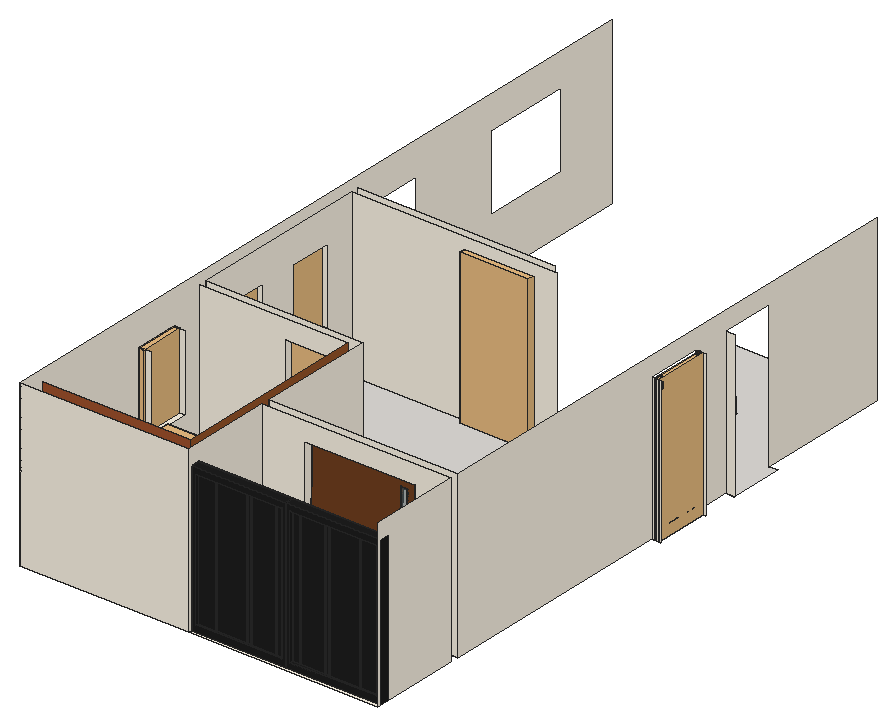
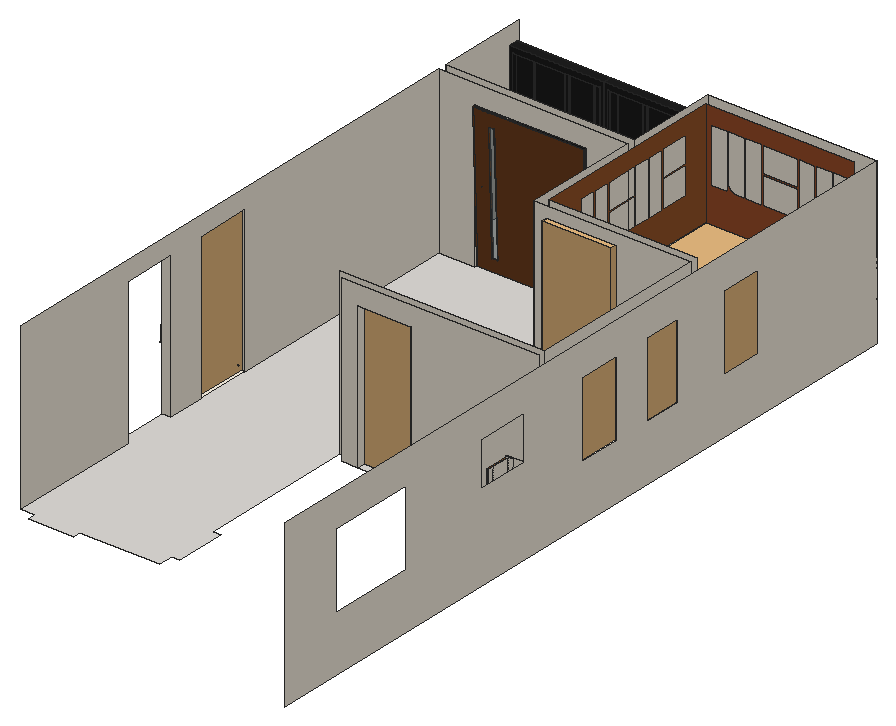
# SketchUp Ruby script. Lengths in inches.
U = 1.inch
M = Sketchup.active_model
def pt(a) = Geom::Point3d.new(a.map { |v| v * U })
def face(e, loops, mat)
  f = e.add_face(loops[0].map { |a| pt(a) })
  loops[1..].each { |l| e.add_face(l.map { |a| pt(a) }).erase! }
  f.material = f.back_material = mat if mat
  f
end
# faces: each face lists its corners as indices into pts; further lists are holes
def faces(e, pts, list, mat = nil) = list.each { |f| face(e, (f[0].is_a?(Array) ? f : [f]).map { |l| l.map { |i| pts[i] } }, mat) }
# xy, xz, yz: faces in a plane at the given z, y or x. An outline is a flat list of corners, or four numbers for a rectangle; further outlines are holes
def ring(l) = l.size == 4 ? [[l[0], l[1]], [l[2], l[1]], [l[2], l[3]], [l[0], l[3]]] : l.each_slice(2).to_a
def flat(e, list, mat, &to3) = list.each { |f| face(e, (f[0].is_a?(Array) ? f : [f]).map { |l| ring(l).map { |u, v| to3.(u, v) } }, mat) }
def xy(e, z, list, mat = nil) = flat(e, list, mat) { |x, y| [x, y, z] }
def xz(e, y, list, mat = nil) = flat(e, list, mat) { |x, z| [x, y, z] }
def yz(e, x, list, mat = nil) = flat(e, list, mat) { |y, z| [x, y, z] }
def lines(e, pts, list) = list.each { |a, b| e.add_line(pt(pts[a]), pt(pts[b])) }
# prism: a flat outline (further loops are holes) pulled along v
def prism(e, loops, v, mat = nil)
  f = face(e, loops, mat); d = Geom::Vector3d.new(v.map { |x| x * U })
  f.pushpull(f.normal.samedirection?(d) ? d.length : -d.length)
end
def box(e, o, s, mat = nil) = prism(e, [[o, [o[0] + s[0], o[1], o[2]], [o[0] + s[0], o[1] + s[1], o[2]], [o[0], o[1] + s[1], o[2]]]], [0, 0, s[2]], mat)
def at(x, y, z, deg = 0) = Geom::Transformation.translation(pt([x, y, z])) * Geom::Transformation.rotation(ORIGIN, Z_AXIS, deg.degrees)
def axes(o, x, y, z) = Geom::Transformation.new([*x, 0, *y, 0, *z, 0, *pt(o).to_a, 1])
def part(name) = M.definitions.add(name)
# library, detail: a bought-in or finely detailed component or shape, given as its bounding box
def library(name, o, s) = part(name).tap { |d| box(d.entities, o, s) }
def detail(e, o, s) = box(e.add_group.entities, o, s)
def put(e, d, t, mat = nil) = e.add_instance(d, t).tap { |i| i.material = mat if mat }
def group(e, t, mat = nil) = e.add_group.tap { |g| g.transformation = t; g.material = mat if mat }.entities
root = M.entities
M.materials.add("Material \#0").color = [86, 53, 35]
M.materials.add("Material \#1").color = [140, 140, 140]
M.materials.add("[0030_OldLace]").color = [253, 245, 230]
M.materials.add("[0040_Peru]").color = [205, 133, 63]
M.materials.add("[0042_Sienna]").color = [160, 82, 45]
M.materials.add("[Color M08]1").color = [30, 30, 30]
M.materials.add("[Metal_Seamed]").color = [118, 119, 115]
M.materials.add("[Terrazzo Tile Accent]").color = [224, 221, 217]
M.materials.add("[Translucent_Glass_Safety]").color = [93, 108, 112]
M.materials["[Translucent_Glass_Safety]"].alpha = 0.5
M.materials.add("[Wood Cherry Original]").color = [152, 86, 42]
M.materials.add("[Wood_Cherry_Original]").color = [112, 63, 31]
M.materials.add("[Wood_Cherry_Original]1").color = [152, 86, 42]
c1 = part("Group\#102")
g1 = group(c1.entities,at(0,0,0))
prism(g1,[[[0,3,72],[70.5,3,72],[70.5,3,0],[0,3,0]],[[67.5,3,3],[67.5,3,69],[3,3,69],[3,3,3]]],[0,-3,0])
c2 = part("Group\#135")
box(c2.entities,[0,0,0],[0.5,1,66])
c3 = part("Framed panel assembly")
g2 = group(c3.entities,at(-446.34,-0.4375,0),"[Color M08]1")
put(g2,c1,axes([69,0,0],[-0.97872,0,0],[0,2.08853,0],[0,0,1.5]))
g3 = group(g2,at(2.9375,4.18,4.5))
g4 = group(g3,at(0,-2.09,0))
box(g4,[0,0,0],[5.39,2.09,99])
box(g4,[49.75,0,0],[13.38,2.09,99])
box(g4,[27.46,0,0],[21.8,2.09,99])
box(g4,[24.13,0,0],[2.84,2.09,99])
box(g4,[5.875,0,0],[17.77,2.09,99])
put(g3,c2,axes([49.26,0,0],[0.97872,0,0],[0,-2.08853,0],[0,0,1.5]))
put(g3,c2,axes([23.65,0,0],[0.97872,0,0],[0,-2.08853,0],[0,0,1.5]))
put(g3,c2,axes([26.97,0,0],[0.97872,0,0],[0,-2.08853,0],[0,0,1.5]))
put(g3,c2,axes([5.39,0,0],[0.97872,0,0],[0,-2.08853,0],[0,0,1.5]))
g5 = group(c3.entities,at(-446.34,-0.4375,0),"[Color M08]1")
put(g5,c1,axes([-69,0,0],[0.97872,0,0],[0,2.08853,0],[0,0,1.5]))
g6 = group(g5,at(-2.9375,4.18,4.5))
g7 = group(g6,at(0,-2.09,0))
box(g7,[-5.39,0,0],[5.39,2.09,99])
box(g7,[-63.13,0,0],[13.38,2.09,99])
box(g7,[-49.26,0,0],[21.8,2.09,99])
box(g7,[-26.97,0,0],[2.84,2.09,99])
box(g7,[-23.65,0,0],[17.77,2.09,99])
put(g6,c2,axes([-49.26,0,0],[-0.97872,0,0],[0,-2.08853,0],[0,0,1.5]))
put(g6,c2,axes([-23.65,0,0],[-0.97872,0,0],[0,-2.08853,0],[0,0,1.5]))
put(g6,c2,axes([-26.97,0,0],[-0.97872,0,0],[0,-2.08853,0],[0,0,1.5]))
put(g6,c2,axes([-5.39,0,0],[-0.97872,0,0],[0,-2.08853,0],[0,0,1.5]))
c4 = library("Group\#25",[0,0,0],[108,114,40.125])
c5 = part("Untitled (1)")
xy(c5.entities,0,[[[-89.01,-44.6,-13.76,84.15],[-78.58,-32.92,-74.95,73.47]]],"[Wood_Cherry_Original]")
xy(c5.entities,2.5,[[-78.58,-32.92,-74.95,73.47]],"[Translucent_Glass_Safety]")
xy(c5.entities,4.25,[[[-89.01,-44.6,-13.76,84.15],[-79.26,-33.6,-74.26,74.15],[-86.22,18.76,-84.6,20.07],[-86.22,-0.43,-84.6,0.51]],[-79.26,-33.6,-74.95,-33.6,-74.95,-32.92,-78.58,-32.92,-78.58,73.47,-74.26,73.47,-74.26,74.15,-79.26,74.15],[-74.95,-33.6,-74.26,73.47]],"[Wood_Cherry_Original]")
xy(c5.entities,5.75,[[-86.22,0.51,-84.6,18.76]],"[Metal_Seamed]")
xy(c5.entities,6.75,[[-86.22,-0.43,-84.6,20.07]],"[Metal_Seamed]")
xz(c5.entities,-44.6,[[-89.01,0,-13.76,4.25]],"[Wood_Cherry_Original]")
xz(c5.entities,-32.92,[[-78.58,0,-74.95,2.5],[-78.58,2.5,-74.95,4.25]],"[Wood_Cherry_Original]")
xz(c5.entities,-0.43,[[-86.22,4.25,-84.6,6.75]],"[Wood_Cherry_Original]")
xz(c5.entities,0.51,[[-86.22,4.25,-84.6,5.75]],"[Metal_Seamed]")
xz(c5.entities,18.76,[[-86.22,4.25,-84.6,5.75]],"[Metal_Seamed]")
xz(c5.entities,20.07,[[-86.22,4.25,-84.6,6.75]],"[Wood_Cherry_Original]")
xz(c5.entities,73.47,[[-78.58,0,-74.95,2.5],[-78.58,2.5,-74.95,4.25]],"[Wood_Cherry_Original]")
xz(c5.entities,84.15,[[-89.01,0,-13.76,4.25]],"[Wood_Cherry_Original]")
yz(c5.entities,-89.01,[[-44.6,0,84.15,4.25]],"[Wood_Cherry_Original]")
yz(c5.entities,-86.22,[[-0.43,4.25,-0.43,6.75,20.07,6.75,20.07,4.25,18.76,4.25,18.76,5.75,0.51,5.75,0.51,4.25]],"[Metal_Seamed]")
yz(c5.entities,-84.6,[[-0.43,4.25,0.51,4.25,0.51,5.75,18.76,5.75,18.76,4.25,20.07,4.25,20.07,6.75,-0.43,6.75]],"[Metal_Seamed]")
yz(c5.entities,-78.58,[[-32.92,2.5,73.47,4.25]],"[Wood_Cherry_Original]")
yz(c5.entities,-78.58,[[-32.92,0,73.47,2.5]],"[Wood_Cherry_Original]1")
yz(c5.entities,-74.95,[[-32.92,0,73.47,2.5],[-32.92,2.5,73.47,4.25]],"[Wood_Cherry_Original]")
yz(c5.entities,-13.76,[[-44.6,0,84.15,4.25]],"[Wood_Cherry_Original]")
c6 = library("Window 82-25",[-14.97,-2.34,0.01],[29.93,4.71,56.48])
c7 = library("Sliding door",[-0.09,-1.01,0],[50.15,5.52,90.11])
c8 = part("3DGeom~18_Defintion")
xz(c8.entities,-241.71,[[-976.3,0,23.7,0,23.7,7.58],[-976.3,0,23.7,7.58,-976.3,7.58]],"Material \#0")
xz(c8.entities,241.71,[[-976.3,0,-976.3,7.58,23.7,7.58],[-976.3,0,23.7,7.58,23.7,0]],"Material \#0")
yz(c8.entities,23.7,[[-241.71,0,0,0,-241.71,7.58],[0,0,0,7.58,-241.71,7.58],[0,0,241.71,0,241.71,7.58],[0,0,241.71,7.58,0,7.58]],"Material \#0")
c9 = part("3DGeom~20_Defintion")
xy(c9.entities,0,[[-976.3,-241.71,-976.3,-223.46,23.7,-241.71],[23.7,-241.71,-976.3,-223.46,5.45,-223.46],[23.7,-241.71,5.45,-223.46,5.45,0],[23.7,-241.71,5.45,0,23.7,0],[-976.3,-223.46,-976.3,-211.85,5.45,-223.46],
  [5.45,-223.46,-976.3,-211.85,-6.16,-211.85],[5.45,-223.46,-6.16,-211.85,-6.16,0],[5.45,-223.46,-6.16,0,5.45,0],[-6.16,0,-6.16,211.85,5.45,223.46],[-6.16,0,5.45,223.46,5.45,0],
  [5.45,0,23.7,241.71,23.7,0],[5.45,0,5.45,223.46,23.7,241.71],[-976.3,211.85,-976.3,223.46,5.45,223.46],[-976.3,211.85,5.45,223.46,-6.16,211.85],[-976.3,223.46,-976.3,241.71,23.7,241.71],
  [-976.3,223.46,23.7,241.71,5.45,223.46]],"Material \#0")
c10 = part("3DGeom~22_Defintion")
xz(c10.entities,-210.625,[[-1016.13,2.47,-1016.13,9.96,-16.28,2.47],[-16.28,2.47,-1016.13,9.96,-16.28,9.96],[-1016.13,9.96,-1016.13,51.7,-16.28,51.7],[-1016.13,9.96,-16.28,51.7,-16.28,9.96],[-1016.13,51.7,-1016.13,72.71,-16.28,51.7]],"Material \#0")
xz(c10.entities,210.625,[[-1016.13,2.47,-16.28,2.47,-1016.13,9.96],[-16.28,2.47,-16.28,9.96,-1016.13,9.96],[-1016.13,9.96,-16.28,51.7,-1016.13,51.7],[-1016.13,9.96,-16.28,9.96,-16.28,51.7],[-1016.13,51.7,-16.28,51.7,-1016.13,72.71]],"Material \#0")
yz(c10.entities,-16.28,[[-210.625,2.47,-210.625,9.96,0,9.96],[-210.625,2.47,0,9.96,0,2.47],[0,2.47,0,9.96,210.625,2.47],[210.625,2.47,0,9.96,210.625,9.96],[-210.625,9.96,-210.625,51.7,0,51.7],
  [-210.625,9.96,0,51.7,0,9.96],[0,9.96,0,51.7,210.625,9.96],[210.625,9.96,0,51.7,210.625,51.7],[-210.625,51.7,0,72.71,0,51.7],[0,51.7,0,72.71,210.625,51.7]],"Material \#0")
p = [[-1016.13,-210.625,72.71],[-16.13,-210.77,73.09],[-16.28,-210.625,51.7],[-16.28,-210.625,51.7],[-16.13,-210.77,73.09],[-16.28,0,72.71],
  [-16.13,210.77,73.09],[-16.28,210.625,51.7],[-16.28,210.625,51.7],[-16.13,210.77,73.09],[-1016.13,210.625,72.71]]
faces(c10.entities,p,[[0,1,2],[3,4,5],[5,6,7],[8,9,10]],"Material \#0")
c11 = part("3DGeom~19_Defintion")
xy(c11.entities,0,[[-6.28,-215.79,-994.45,-208.55,-13.52,-208.55],[-994.45,-215.79,-994.45,-208.55,-6.28,-215.79],[-6.28,-215.79,-13.52,-208.55,-13.52,0],[-6.28,-215.79,-13.52,0,-6.28,0],[-13.52,0,-13.52,208.55,-6.28,215.79],
  [-13.52,0,-6.28,215.79,-6.28,0],[-994.45,208.55,-6.28,215.79,-13.52,208.55],[-994.45,208.55,-994.45,215.79,-6.28,215.79]],"Material \#0")
p = [[-13.52,-208.55,0],[-994.45,-208.55,0],[-994.45,-207.81,0.07],[-14.25,-207.81,0.07],[-13.52,-208.55,0],[-14.25,-207.81,0.07],
  [-14.25,0,0.07],[-13.52,0,0],[-13.52,208.55,0],[-14.25,207.81,0.07],[-13.52,208.55,0],[-14.25,207.81,0.07],
  [-994.45,207.81,0.07],[-994.45,208.55,0],[-994.45,-207.21,0.27],[-994.45,-207.21,0.27],[-14.86,-207.21,0.27],[-14.86,-207.21,0.27],
  [-14.86,0,0.27],[-14.86,0,0.27],[-14.86,0,0.27],[-14.86,0,0.27],[-14.86,207.21,0.27],[-14.86,207.21,0.27],
  [-994.45,207.21,0.27],[-994.45,207.21,0.27],[-14.86,-207.21,0.27],[-994.45,-207.21,0.27],[-994.45,-206.74,0.6],[-15.33,-206.74,0.6],
  [-14.86,-207.21,0.27],[-15.33,-206.74,0.6],[-15.33,0,0.6],[-14.86,0,0.27],[-14.86,207.21,0.27],[-15.33,206.74,0.6],
  [-14.86,207.21,0.27],[-15.33,206.74,0.6],[-994.45,206.74,0.6],[-994.45,207.21,0.27],[-994.45,-206.4,1.07],[-15.66,-206.4,1.07],
  [-15.66,-206.4,1.07],[-15.66,0,1.07],[-15.66,206.4,1.07],[-15.66,206.4,1.07],[-994.45,206.4,1.07],[-994.45,-206.2,1.68],
  [-15.86,-206.2,1.68],[-15.86,-206.2,1.68],[-15.86,0,1.68],[-15.86,206.2,1.68],[-15.86,206.2,1.68],[-994.45,206.2,1.68],
  [-994.45,-206.13,2.41],[-15.93,-206.13,2.41],[-15.93,-206.13,2.41],[-15.93,0,2.41],[-15.93,206.13,2.41],[-15.93,206.13,2.41],
  [-994.45,206.13,2.41],[-994.45,-206.13,71.16],[-994.45,-206.22,71.59],[-15.79,-206.28,71.53],[-15.79,-206.28,71.53],[-15.84,0,71.59],
  [-15.93,0,71.16],[-15.79,206.28,71.53],[-15.79,206.28,71.53],[-994.45,206.22,71.59],[-994.45,206.13,71.16],[-15.79,-206.28,71.53],
  [-994.45,-206.48,71.84],[-994.45,-206.9,71.93],[-15.16,-206.9,71.93],[-15.79,-206.28,71.53],[-15.79,-206.28,71.53],[-15.16,-206.9,71.93],
  [-15.16,0,71.93],[-994.45,-206.48,71.84],[-15.59,0,71.84],[-15.79,-206.28,71.53],[-15.59,0,71.84],[-15.79,206.28,71.53],
  [-15.16,206.9,71.93],[-15.59,0,71.84],[-15.79,206.28,71.53],[-994.45,206.48,71.84],[-15.79,206.28,71.53],[-15.16,206.9,71.93],
  [-994.45,206.9,71.93],[-994.45,206.48,71.84],[-15.79,206.28,71.53],[-994.45,-227.27,72.01],[5.41,-227.47,72.33],[4.78,-226.84,71.93],
  [4.78,-226.84,71.93],[5.41,-227.47,72.33],[5.21,0,72.01],[-994.45,-226.84,71.93],[-994.45,-227.27,72.01],[5.21,0,72.01],
  [4.78,0,71.93],[4.78,226.84,71.93],[5.21,0,72.01],[5.21,0,72.01],[5.41,227.47,72.33],[4.78,226.84,71.93],
  [5.41,227.47,72.33],[-994.45,227.27,72.01],[-994.45,227.27,72.01],[-994.45,226.84,71.93],[-994.45,-227.27,72.01],[-994.45,-227.53,72.27],
  [5.41,-227.47,72.33],[5.41,-227.47,72.33],[5.47,0,72.27],[5.21,0,72.01],[5.41,227.47,72.33],[5.41,227.47,72.33],
  [-994.45,227.53,72.27],[-994.45,227.27,72.01],[-994.45,-227.61,72.7],[-994.45,-227.61,74.4375],[-994.45,-227.61,74.4375],[5.55,-227.61,74.4375],
  [5.55,-227.61,74.4375],[5.55,0,74.4375],[5.55,0,72.7],[5.55,227.61,74.4375],[5.55,227.61,74.4375],[-994.45,227.61,74.4375],
  [-994.45,227.61,74.4375],[-994.45,227.61,72.7]]
faces(c11.entities,p,[[0,1,2],[2,3,0],[4,5,6],[6,7,4],[8,7,6],[6,9,8],[10,11,12],[12,13,10],
  [3,2,14],[15,16,3],[5,17,18],[19,6,5],[9,6,20],[21,22,9],[11,23,24],[25,12,11],
  [26,27,28],[28,29,26],[30,31,32],[32,33,30],[34,33,32],[32,35,34],[36,37,38],[38,39,36],
  [29,28,40],[40,41,29],[31,42,43],[43,32,31],[35,32,43],[43,44,35],[37,45,46],[46,38,37],
  [41,40,47],[47,48,41],[42,49,50],[50,43,42],[44,43,50],[50,51,44],[45,52,53],[53,46,45],
  [48,47,54],[54,55,48],[49,56,57],[57,50,49],[51,50,57],[57,58,51],[52,59,60],[60,53,52],
  [61,62,63],[64,65,66],[66,65,67],[68,69,70],[71,72,73],[73,74,75],[76,77,78],[62,79,63],
  [78,80,76],[81,82,65],[83,80,78],[78,84,83],[65,85,86],[68,87,69],[88,89,90],[90,91,92],
  [93,94,95],[96,97,98],[95,99,100],[101,102,96],[103,102,104],[105,106,103],[107,108,109],[110,111,107],
  [112,113,114],[115,116,117],[117,116,118],[119,120,121],[114,122,123],[124,125,114],[113,122,114],[115,126,127],
  [127,128,115],[115,128,116],[118,128,127],[127,129,118],[116,128,118],[119,130,131],[132,133,119],[119,133,120]],"Material \#0")
c12 = part("3DGeom~15_Defintion")
xy(c12.entities,0,[[-961.58,-251.9,-958.5,-248.8125,-961.58,-237.8],[-961.58,-251.9,28.8,-248.8125,-958.5,-248.8125],[-961.58,-251.9,36.25,-251.9,28.8,-248.8125],[36.25,-251.9,19.98,-239.99,28.8,-248.8125],[36.25,-251.9,22.16,-237.8,19.98,-239.99],
  [-958.5,-248.8125,-958.5,-237.8,-961.58,-237.8],[19.98,-239.99,22.16,-237.8,3.36,-223.37],[-958.5,-237.8,-958.5,-223.37,-961.58,-220.28],[-961.58,-237.8,-958.5,-237.8,-961.58,-220.28],[22.16,-237.8,4.64,-220.28,3.36,-223.37],
  [-958.5,-223.37,4.64,-220.28,-961.58,-220.28],[-958.5,-223.37,3.36,-223.37,4.64,-220.28],[5.29,-219.63,8.375,-218.35,5.29,0],[8.375,-218.35,8.375,0,5.29,0],[5.29,0,8.375,0,5.29,219.63],
  [8.375,0,8.375,218.35,5.29,219.63],[8.375,218.35,22.8125,237.15,5.29,219.63],[-961.58,220.28,-958.5,223.37,-961.58,237.8],[-961.58,220.28,3.36,223.37,-958.5,223.37],[-961.58,220.28,4.64,220.28,3.36,223.37],
  [4.64,220.28,19.98,239.99,3.36,223.37],[4.64,220.28,22.16,237.8,19.98,239.99],[-958.5,223.37,-958.5,237.8,-961.58,237.8],[-958.5,237.8,-958.5,248.8125,-961.58,251.9],[-961.58,237.8,-958.5,237.8,-961.58,251.9],
  [22.16,237.8,28.8,248.8125,19.98,239.99],[22.16,237.8,36.25,251.9,28.8,248.8125],[-958.5,248.8125,36.25,251.9,-961.58,251.9],[-958.5,248.8125,28.8,248.8125,36.25,251.9]],"Material \#0")
xy(c12.entities,7.48,[[-962.79,-238.36,23.37,-238.36,-962.79,-219.67],[23.37,-238.36,4.67,-219.67,-962.79,-219.67],[23.37,-238.36,23.37,0,4.67,-219.67],[4.67,-219.67,23.37,0,4.67,0],[23.37,0,23.37,238.36,4.67,219.67],
  [4.67,0,23.37,0,4.67,219.67],[-962.79,219.67,23.37,238.36,-962.79,238.36],[-962.79,219.67,4.67,219.67,23.37,238.36]],"Material \#0")
xy(c12.entities,63.5625,[[-962.79,-238.36,-962.79,-219.67,4.67,-219.67],[-962.79,-238.36,4.67,-219.67,23.37,-238.36],[23.37,-238.36,4.67,-219.67,23.37,0],[4.67,-219.67,4.67,0,23.37,0],[23.37,0,4.67,219.67,23.37,238.36],
  [4.67,0,4.67,219.67,23.37,0],[-962.79,219.67,-962.79,238.36,4.67,219.67],[4.67,219.67,-962.79,238.36,23.37,238.36]],"Material \#0")
xy(c12.entities,69.64,[[-962.79,-219.62,4.63,-219.62,-962.79,-200.32],[4.63,-219.62,-14.68,-200.32,-962.79,-200.32],[4.63,-219.62,4.63,0,-14.68,-200.32],[-14.68,-200.32,4.63,0,-14.68,0],[-14.68,0,4.63,0,-14.68,200.32],
  [4.63,0,4.63,219.62,-14.68,200.32],[-962.79,200.32,-14.68,200.32,4.63,219.62],[-962.79,200.32,4.63,219.62,-962.79,219.62]],"Material \#0")
xy(c12.entities,71.04,[[-961.58,-251.9,-958.5,-248.8125,28.8,-248.8125],[-961.58,-251.9,-961.58,-237.8,-958.5,-248.8125],[-961.58,-251.9,28.8,-248.8125,36.25,-251.9],[36.25,-251.9,19.98,-239.99,22.16,-237.8],[36.25,-251.9,28.8,-248.8125,19.98,-239.99],
  [-958.5,-248.8125,-961.58,-237.8,-958.5,-237.8],[19.98,-239.99,3.36,-223.37,22.16,-237.8],[-958.5,-237.8,-961.58,-220.28,-958.5,-223.37],[-961.58,-237.8,-961.58,-220.28,-958.5,-237.8],[22.16,-237.8,3.36,-223.37,4.64,-220.28],
  [-958.5,-223.37,-961.58,-220.28,4.64,-220.28],[-958.5,-223.37,4.64,-220.28,3.36,-223.37],[5.29,-219.63,5.29,0,8.375,-218.35],[8.375,-218.35,5.29,0,8.375,0],[5.29,0,5.29,219.63,8.375,0],
  [8.375,0,5.29,219.63,8.375,218.35],[8.375,218.35,5.29,219.63,22.8125,237.15],[-961.58,220.28,-958.5,223.37,3.36,223.37],[-961.58,220.28,-961.58,237.8,-958.5,223.37],[-961.58,220.28,3.36,223.37,4.64,220.28],
  [4.64,220.28,3.36,223.37,19.98,239.99],[4.64,220.28,19.98,239.99,22.16,237.8],[-958.5,223.37,-961.58,237.8,-958.5,237.8],[-958.5,237.8,-961.58,251.9,-958.5,248.8125],[-961.58,237.8,-961.58,251.9,-958.5,237.8],
  [22.16,237.8,19.98,239.99,28.8,248.8125],[22.16,237.8,28.8,248.8125,36.25,251.9],[-958.5,248.8125,-961.58,251.9,36.25,251.9],[-958.5,248.8125,36.25,251.9,28.8,248.8125]],"Material \#0")
xz(c12.entities,-238.36,[[-962.79,63.5625,23.37,63.5625,23.37,72.07],[-962.79,63.5625,23.37,72.07,-962.79,72.07]],"Material \#0")
xz(c12.entities,-219.67,[[-962.79,7.48,4.67,7.48,-962.79,63.5625],[4.67,7.48,4.67,63.5625,-962.79,63.5625]],"Material \#0")
xz(c12.entities,219.67,[[-962.79,7.48,-962.79,63.5625,4.67,7.48],[4.67,7.48,-962.79,63.5625,4.67,63.5625]],"Material \#0")
xz(c12.entities,238.36,[[-962.79,63.5625,-962.79,72.07,23.37,72.07],[-962.79,63.5625,23.37,72.07,23.37,63.5625]],"Material \#0")
yz(c12.entities,4.67,[[-219.67,7.48,0,7.48,-219.67,63.5625],[0,7.48,0,63.5625,-219.67,63.5625],[0,7.48,219.67,63.5625,0,63.5625],[0,7.48,219.67,7.48,219.67,63.5625]],"Material \#0")
yz(c12.entities,23.37,[[-238.36,63.5625,0,63.5625,-238.36,72.07],[0,63.5625,0,72.07,-238.36,72.07],[0,63.5625,238.36,63.5625,238.36,72.07],[0,63.5625,238.36,72.07,0,72.07]],"Material \#0")
p = [[36.9,-251.24,0],[37.21,0,-0.16],[34.125,0,-0.14],[36.9,251.24,0],[33.83,243.81,0.02],[33.83,-243.8,0.02],
  [22.8125,-237.15,0],[24.99,-234.97,-0.01],[5.375,-220.37,0],[23.37,-238.36,7.48],[4.67,-219.67,7.48],[4.67,-219.67,7.48],
  [23.37,-238.36,7.48],[23.37,-238.36,0],[4.67,-219.67,7.48],[23.37,-238.36,0],[5.375,-220.37,0],[5.375,-220.37,0],
  [23.37,-238.36,0],[5.29,-219.63,0],[8.375,-218.35,0],[-15.36,-199.64,1.62],[4.67,-219.67,7.48],[5.375,-220.37,0],
  [-13.8,-201.19,0.06],[5.375,-220.37,0],[5.375,-220.37,0],[-14.84,-200.15,0.58],[5.375,-220.37,0],[-13.8,-201.19,0.06],
  [-6.08,-208.92,0],[5.375,-220.37,0],[-13.8,-201.19,0.06],[-6.08,-208.92,0],[-13.8,-201.19,0.06],[5.375,-220.37,0],
  [-6.08,-208.92,0],[-13.8,-201.19,0.06],[-13.09,-201.91,0],[-6.08,-208.92,0],[-13.09,-201.91,0],[-13.8,-201.19,0.06],
  [-15.36,199.64,1.62],[4.67,219.67,7.48],[5.375,220.37,0],[-13.8,201.19,0.06],[5.375,220.37,0],[5.375,220.37,0],
  [4.67,219.67,7.48],[-14.84,200.15,0.58],[5.375,220.37,0],[-13.8,201.19,0.06],[-6.08,208.92,0],[-13.09,201.91,0],
  [-13.8,201.19,0.06],[-6.08,208.92,0],[-13.8,201.19,0.06],[5.375,220.37,0],[-6.08,208.92,0],[5.375,220.37,0],
  [-13.8,201.19,0.06],[-6.08,208.92,0],[-13.8,201.19,0.06],[-13.09,201.91,0],[8.375,218.35,0],[24.99,234.97,-0.01],
  [22.8125,237.15,0],[23.37,238.36,7.48],[23.37,238.36,0],[23.37,238.36,0],[5.375,220.37,0],[5.375,220.37,0],
  [23.37,238.36,7.48],[4.67,219.67,7.48],[5.375,220.37,0],[23.37,238.36,0],[23.37,238.36,7.48],[-13.8,-201.19,0.06],
  [-14.84,-200.15,0.58],[-14.38,-200.61,0.26],[-13.8,-201.19,0.06],[-13.8,-201.19,0.06],[-14.38,-200.61,0.26],[-13.8,201.19,0.06],
  [-14.84,200.15,0.58],[-13.8,201.19,0.06],[-14.38,200.61,0.26],[-14.38,200.61,0.26],[-13.8,201.19,0.06],[4.63,-219.62,69.64],
  [4.63,-219.62,69.64],[-15.42,-199.57,9.43],[-15.36,-199.64,1.62],[-15.16,-199.83,1.04],[-15.16,-199.83,1.04],[-15.16,199.83,1.04],
  [-15.36,199.64,1.62],[-15.16,199.83,1.04],[-15.42,199.57,9.43],[4.63,219.62,69.64],[4.67,219.67,7.48],[4.63,219.62,69.64],
  [4.63,-219.62,69.64],[4.67,-219.67,63.5625],[4.67,-219.67,63.5625],[4.67,-219.67,7.48],[-15.28,-199.71,69.25],[4.63,-219.62,69.64],
  [-15.42,-199.57,9.43],[-15.28,-199.71,69.25],[-15.42,-199.57,2.34],[-15.42,-199.57,2.34],[-15.42,199.57,2.34],[-15.42,199.57,9.43],
  [-15.28,199.71,69.25],[-15.28,199.71,69.25],[4.63,219.62,69.64],[4.63,219.62,69.64],[4.67,219.67,63.5625],[4.67,219.67,63.5625],
  [-15.42,199.57,2.34],[4.67,-219.67,63.5625],[4.63,-219.62,69.64],[4.67,219.67,7.48],[4.67,219.67,63.5625],[4.63,219.62,69.64],
  [4.63,-219.62,69.64],[-15.28,-199.71,69.25],[-15.28,-199.71,69.25],[-15.42,-199.57,48.99],[-15.42,-199.57,48.99],[-15.28,-199.71,69.25],
  [-15.42,199.57,48.99],[-15.28,199.71,69.25],[-15.28,199.71,69.25],[-15.42,199.57,48.99],[4.63,219.62,69.64],[4.63,-219.62,69.64],
  [23.37,-238.36,72.07],[4.67,-219.67,63.5625],[4.67,-219.67,63.5625],[23.37,-238.36,63.5625],[23.37,-238.36,72.07],[4.67,-219.67,63.5625],
  [5.24,-220.23,70.03],[23.37,-238.36,72.07],[23.37,-238.36,63.5625],[4.67,-219.67,63.5625],[4.67,-219.67,63.5625],[4.63,-219.62,69.64],
  [4.63,219.62,69.64],[23.37,238.36,72.07],[4.67,219.67,63.5625],[4.67,219.67,63.5625],[5.24,220.23,70.03],[4.63,219.62,69.64],
  [23.37,238.36,63.5625],[4.67,219.67,63.5625],[4.67,219.67,63.5625],[23.37,238.36,63.5625],[23.37,238.36,72.07],[4.67,219.67,63.5625],
  [23.37,238.36,72.07],[4.63,-219.62,69.64],[-14.68,-200.32,69.64],[-15.28,-199.71,69.25],[-15.28,-199.71,69.25],[-14.68,-200.32,69.64],
  [4.63,-219.62,69.64],[-15.28,199.71,69.25],[-14.68,200.32,69.64],[4.63,219.62,69.64],[4.63,219.62,69.64],[-14.68,200.32,69.64],
  [4.63,-219.62,69.64],[5.24,-220.23,70.03],[23.37,-238.36,72.07],[4.63,219.62,69.64],[5.24,220.23,70.03],[5.375,-220.37,72.07],
  [5.375,-220.37,72.07],[23.37,-238.36,72.07],[5.375,220.37,72.07],[23.37,238.36,72.07],[5.375,220.37,72.07],[33.83,-243.8,71.03],
  [36.9,-251.24,71.04],[22.8125,-237.15,71.04],[34.125,0,71.19],[37.21,0,71.2],[24.99,-234.97,71.05],[5.29,-219.63,71.04],
  [8.375,-218.35,71.04],[33.83,243.81,71.03],[36.9,251.24,71.04],[22.8125,237.15,71.04],[24.99,234.97,71.05],[8.375,218.35,71.04]]
faces(c12.entities,p,[[0,1,2],[1,3,4],[4,2,1],[2,5,0],[6,0,5],[5,7,6],[8,9,10],[11,12,13],
  [14,15,16],[17,18,9],[19,6,7],[7,20,19],[21,22,23],[24,21,25],[26,10,27],[28,27,29],
  [30,31,32],[33,34,35],[36,37,38],[39,40,41],[42,43,44],[45,42,46],[47,48,49],[50,49,51],
  [52,53,54],[55,56,57],[58,59,60],[61,62,63],[64,65,66],[43,67,68],[43,69,70],[71,72,73],
  [74,75,76],[3,66,65],[65,4,3],[77,78,21],[27,79,80],[81,82,78],[83,84,42],[85,86,84],
  [49,87,88],[10,89,27],[90,91,27],[92,93,27],[91,92,27],[78,94,21],[84,95,42],[96,97,49],
  [98,96,49],[99,98,49],[100,101,49],[21,102,103],[21,104,105],[21,106,107],[21,108,109],[91,110,92],
  [21,111,108],[42,112,113],[42,113,114],[42,115,116],[42,117,118],[42,119,43],[98,120,96],[10,121,122],
  [123,124,125],[126,127,91],[128,129,91],[108,130,131],[113,132,133],[134,135,98],[136,134,98],[137,138,139],
  [140,141,142],[143,142,144],[145,146,147],[148,144,149],[150,151,152],[153,154,155],[151,156,157],[158,159,160],
  [161,162,154],[163,164,165],[166,167,168],[169,170,171],[172,173,134],[174,175,176],[177,178,151],[142,179,144],
  [175,180,181],[178,182,151],[183,184,154],[185,186,187],[186,185,188],[188,189,186],[187,190,185],[190,187,191],
  [191,192,190],[189,188,193],[193,194,189],[195,196,197],[196,195,194],[194,193,196]],"Material \#0")
c13 = library("3DGeom~16_Defintion",[-962.62,-252.34,-11.22],[1000,504.68,93.46])
xy(root,0,[[123,4.46,261,13.46],[261,254.14,267,294.63]],"[0030_OldLace]")
xy(root,0,[[123,13.46,261,13.46,261,71.46,234.43,71.46,234.43,77.46,261,77.46,261,321.88,267,321.88,267,361.78,261,361.78,261,459.46,250.125,459.46,250.125,465.46,217.25,465.46,217.25,459.46,159,459.46,159,449.03,153,449.03,153,411.21,159,411.21,159,295.46,140.9375,295.46,140.9375,301.46,102,301.46,102,295.46,9,295.46,9,162.9,71.67,162.9,71.67,157.46,106.375,157.46,106.375,162.9,123,162.9,123,77.46,153.875,77.46,153.875,71.46,123,71.46]],"[Terrazzo Tile Accent]")
xy(root,2.4375,[[31.28,302.96,32.22,314.96],[31.28,315.46,32.22,319.46]],"[0030_OldLace]")
xy(root,41,[[0,112.59,9,143.46],[0,185.34,9,214.09],[0,241.59,9,273.53]],"[0030_OldLace]")
xy(root,45.1875,[[31.28,302.96,32.22,314.96]],"[0040_Peru]")
xy(root,45.1875,[[31.28,315.46,32.22,319.46]],"[Wood Cherry Original]")
xz(root,4.46,[[0,0,123,120]],"[0030_OldLace]")
xz(root,13.46,[[[9,42.3125,117,120],[49.875,67.6875,76,87.9375],[49.875,88.4375,76,107.625],[101.5,67.6875,113.5,107.625],[76.5,67.6875,88.5,107.625],[37.375,67.6875,49.375,107.625],[24.875,67.6875,36.875,107.625],[12.375,67.6875,24.375,107.625],[89,67.6875,95,67.6875,96.4,67.85,97.73,68.33,98.91,69.1,99.875,70.12,100.59,71.34,101,72.6875,101,107.6875,89,107.6875]]],"[0042_Sienna]")
xz(root,71.46,[[123,0,153.875,0,153.875,106,234.43,106,234.43,0,261,0,261,120,123,120]],"[0030_OldLace]")
xz(root,77.46,[[123,0,123,120,261,120,261,0,234.43,0,234.43,106,153.875,106,153.875,0]],"[0030_OldLace]")
xz(root,112.59,[[0,41,9,96]],"[0030_OldLace]")
xz(root,143.46,[[0,41,9,96]],"[0030_OldLace]")
xz(root,157.46,[[9,0,71.67,0,71.67,106,106.375,106,106.375,0,117,0,117,120,9,120]],"[0030_OldLace]")
xz(root,162.9,[[9,0,9,120,123,120,123,0,106.375,0,106.375,106,71.67,106,71.67,0]],"[0030_OldLace]")
xz(root,185.34,[[0,41,9,96]],"[0030_OldLace]")
xz(root,214.09,[[0,41,9,96]],"[0030_OldLace]")
xz(root,241.59,[[0,41,9,96]],"[0030_OldLace]")
xz(root,254.14,[[261,0,268.125,106]],"[0030_OldLace]")
xz(root,273.53,[[0,41,9,96]],"[0030_OldLace]")
xz(root,294.63,[[261,0,268.125,106]],"[0030_OldLace]")
xz(root,295.46,[[9,0,102,0,102,106,140.9375,106,140.9375,0,159,0,159,120,9,120]],"[0030_OldLace]")
xz(root,301.46,[[27.65,0,27.65,1.9375,31.28,1.9375,31.28,45.6875,32.64,45.6875,32.64,46.625,9,46.625,9,120,153,120,153,0,140.9375,0,140.9375,106,102,106,102,0],[9,0,27.65,1.9375],[9,1.9375,27.65,46.625],[27.65,1.9375,31.28,45.6875],[27.65,45.6875,32.64,46.625]],"[0030_OldLace]")
xz(root,302.96,[[31.28,2.4375,32.22,45.1875]],"[0040_Peru]")
xz(root,314.96,[[31.28,2.4375,32.22,45.1875]],"[0040_Peru]")
xz(root,315.46,[[31.28,2.4375,32.22,45.1875]],"[Wood Cherry Original]")
xz(root,319.46,[[31.28,2.4375,32.22,45.1875]],"[Wood Cherry Original]")
xz(root,321.88,[[261,0,267.4375,106]],"[0030_OldLace]")
yz(root,0,[[[4.46,0,544.46,120],[434.03,41,497.9,96],[241.59,41,273.53,96],[112.59,41,143.46,96],[185.34,41,214.09,96],[326.03,63.5,365.53,96]]],"[0030_OldLace]")
yz(root,9,[[[162.9,0,295.46,120],[241.59,41,273.53,96],[185.34,41,214.09,96]],[108.71,2.1875,111.18,42.3125]],"[0030_OldLace]")
yz(root,31.28,[[302.96,2.4375,314.96,45.1875],[315.46,2.4375,319.46,45.1875]],"[0030_OldLace]")
yz(root,32.22,[[302.96,2.4375,314.96,45.1875]],"[0040_Peru]")
yz(root,32.22,[[315.46,2.4375,319.46,45.1875]],"[Wood Cherry Original]")
yz(root,71.67,[[157.46,0,162.9,106]],"[0030_OldLace]")
yz(root,102,[[295.46,0,301.46,106]],"[0030_OldLace]")
yz(root,106.375,[[157.46,0,162.9,106]],"[0030_OldLace]")
yz(root,117,[[13.46,0,13.46,42.3125,127.47,42.3125,127.47,2.1875,127.59,2.1875,127.59,0]],"[0030_OldLace]")
yz(root,117,[[[127.59,0,127.59,2.1875,127.47,2.1875,127.47,42.3125,13.46,42.3125,13.46,120,157.46,120,157.46,0],[78.78,67.8125,102.78,88.125],[115.78,67.8125,127.78,107.6875],[103.28,67.8125,115.28,107.6875],[66.28,67.8125,78.28,107.6875],[53.78,67.8125,65.78,107.6875],[78.78,88.625,102.78,107.6875],[32.34,67.8125,53.28,88.125],[32.34,88.625,53.28,107.6875]]],"[Wood Cherry Original]")
yz(root,123,[[4.46,0,71.46,120],[77.46,0,162.9,120]],"[0030_OldLace]")
yz(root,140.9375,[[295.46,0,301.46,106]],"[0030_OldLace]")
yz(root,153.875,[[71.46,0,77.46,106]],"[0030_OldLace]")
yz(root,234.43,[[71.46,0,77.46,106]],"[0030_OldLace]")
yz(root,261,[[4.46,0,71.46,120],[77.46,0,77.46,120,459.46,120,459.46,0,361.78,0,361.78,106,321.88,106,321.88,0,294.63,0,294.63,106,254.14,106,254.14,0]],"[0030_OldLace]")
yz(root,263.95,[[327.85,50.7,327.75,50.79,327.76,50.8],[327.75,50.79,327.68,50.89,327.6875,50.9],[327.75,50.79,327.6875,50.9,327.76,50.8],[327.68,50.89,327.61,51.02,327.62,51.02],[327.68,50.89,327.62,51.02,327.6875,50.9],
  [327.61,51.02,327.5625,51.15,327.57,51.16],[327.61,51.02,327.57,51.16,327.62,51.02],[327.5625,51.15,327.53,51.3,327.54,51.3],[327.5625,51.15,327.54,51.3,327.57,51.16],[327.53,51.3,327.52,51.46,327.53,51.46],
  [327.53,51.3,327.53,51.46,327.54,51.3],[327.52,51.46,327.52,61.35,327.53,61.35],[327.52,51.46,327.53,61.35,327.53,51.46]],"Material \#1")
yz(root,264.1,[[327.85,50.7,327.76,50.8,327.75,50.79],[327.75,50.79,327.6875,50.9,327.68,50.89],[327.75,50.79,327.76,50.8,327.6875,50.9],[327.68,50.89,327.62,51.02,327.61,51.02],[327.68,50.89,327.6875,50.9,327.62,51.02],
  [327.61,51.02,327.57,51.16,327.5625,51.15],[327.61,51.02,327.62,51.02,327.57,51.16],[327.5625,51.15,327.54,51.3,327.53,51.3],[327.5625,51.15,327.57,51.16,327.54,51.3],[327.53,51.3,327.53,51.46,327.52,51.46],
  [327.53,51.3,327.54,51.3,327.53,51.46],[327.52,51.46,327.53,51.46,327.53,61.35],[327.52,51.46,327.53,61.35,327.52,61.35]],"Material \#1")
yz(root,265.64,[[260.02,50.95,259.95,51.08,259.96,51.08],[259.95,51.08,259.9,51.21,259.91,51.22],[259.95,51.08,259.91,51.22,259.96,51.08],[259.9,51.21,259.87,51.36,259.88,51.36],[259.9,51.21,259.88,51.36,259.91,51.22],
  [259.87,51.36,259.86,51.52,259.87,51.52],[259.87,51.36,259.87,51.52,259.88,51.36],[259.86,51.52,259.86,61.42,259.87,61.41],[259.86,51.52,259.87,61.41,259.87,51.52],[261.16,53.65,261.16,61.41,261.17,61.42]],"Material \#1")
p = [[9,108.71,0],[9,34.78,0],[9,108.71,2.1875],[29.25,111.18,2.1875],[29.25,35.9,2.1875],[9,35.9,42.3125],
  [9,108.71,42.3125],[31.8125,111.18,2.1875],[31.8125,35.9,2.1875],[26.375,108.71,0],[117,127.59,0],[98.6875,127.59,0],
  [98.6875,34.21,0],[26.375,34.78,0],[9,13.46,0],[117,13.46,0],[26.375,34.21,0]]
lines(root,p,[[0,1],[0,2],[3,4],[5,6],[7,8],[3,7],[9,0],[10,11],[12,11],[13,9],[14,15],[12,16]])
put(root,c3,at(638.34,7.39,0))
put(root,c4,at(9,13.46,2.1875),"[0030_OldLace]")
g8 = group(root,at(9,13.46,0),"[0030_OldLace]")
xy(g8,2.1875,[[0,0,108,0,108,114.125,89.6875,114.125,89.6875,20.75,17.375,20.75,17.375,95.25,0,95.25]])
xz(g8,20.75,[[17.375,0,89.6875,2.1875]])
xz(g8,95.25,[[0,0,17.375,2.1875]])
xz(g8,114.125,[[89.6875,0,108,2.1875]])
yz(g8,17.375,[[20.75,0,95.25,2.1875]])
yz(g8,89.6875,[[20.75,0,114.125,2.1875]])
put(root,c5,axes([139.1875,78.13,69.05],[-1.07,0,0],[0,-0.02872,-0.8223],[0,-0.14991,0.00523]))
g9 = group(root,at(9,13.46,0),"[0030_OldLace]")
p = [[108,144,0],[97.375,144,0],[108,0,0],[0,144,0],[0,0,0],[62.67,144,0]]
lines(g9,p,[[0,1],[2,0],[3,4],[5,3],[1,5],[4,2]])
put(root,c6,axes([2.68,127.8125,39.44],[0,-1.1024,0],[0.85,0,0],[0,0,1]))
put(root,c7,axes([63.63,162.92,0.33],[1,0,0],[0,1,0],[0,0,1.2376]))
put(root,c6,axes([3.08,199.3125,39.44],[0,-1.04815,0],[0.68,0,0],[0,0,1]))
put(root,c6,axes([3.08,257.97,39.44],[0,-1.12152,0],[0.68,0,0],[0,0,1]))
put(root,c8,axes([263.98,274.39,3.96],[0,0,-0.10451],[0,0.07911,0],[0.03,0,0]),"Material \#0")
put(root,c9,axes([263.98,274.39,3.96],[0,0,-0.10451],[0,0.07911,0],[0.03,0,0]),"Material \#0")
put(root,c10,axes([263.98,274.39,3.96],[0,0,-0.10042],[0,0.07601,0],[0.02882,0,0]),"Material \#0")
put(root,c11,axes([263.98,274.39,3.96],[0,0,-0.10261],[0,0.07766,0],[0.02945,0,0]),"Material \#0")
put(root,c12,axes([263.98,274.39,3.96],[0,0,-0.10598],[0,0.08022,0],[0.03042,0,0]),"Material \#0")
put(root,c13,axes([263.98,274.39,3.96],[0,0,-0.106],[0,0.08023,0],[0.03042,0,0]),"Material \#0")
put(root,c7,axes([141.76,295.28,0.33],[-1,0,0],[0,-1,0],[0,0,1.2376]))
